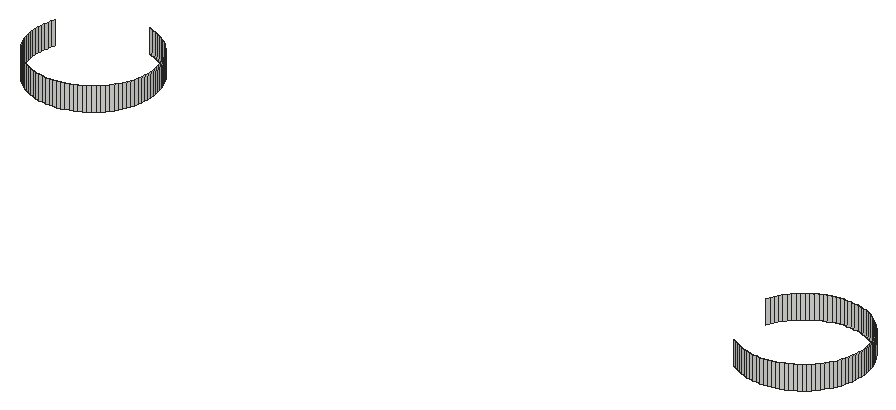
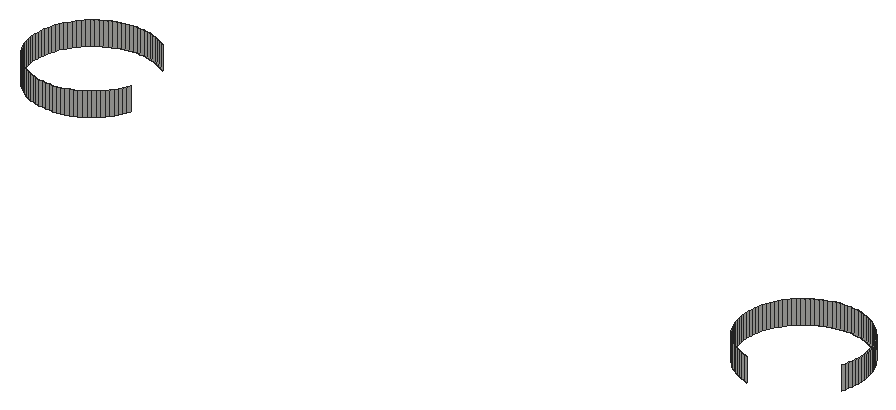
# SketchUp Ruby script. Lengths in inches.
U = 1.inch
M = Sketchup.active_model
def pt(a) = Geom::Point3d.new(a.map { |v| v * U })
def face(e, loops, mat)
  f = e.add_face(loops[0].map { |a| pt(a) })
  loops[1..].each { |l| e.add_face(l.map { |a| pt(a) }).erase! }
  f.material = f.back_material = mat if mat
  f
end
# faces: each face lists its corners as indices into pts; further lists are holes
def faces(e, pts, list, mat = nil) = list.each { |f| face(e, (f[0].is_a?(Array) ? f : [f]).map { |l| l.map { |i| pts[i] } }, mat) }
# xy, xz, yz: faces in a plane at the given z, y or x. An outline is a flat list of corners, or four numbers for a rectangle; further outlines are holes
def ring(l) = l.size == 4 ? [[l[0], l[1]], [l[2], l[1]], [l[2], l[3]], [l[0], l[3]]] : l.each_slice(2).to_a
def flat(e, list, mat, &to3) = list.each { |f| face(e, (f[0].is_a?(Array) ? f : [f]).map { |l| ring(l).map { |u, v| to3.(u, v) } }, mat) }
def xy(e, z, list, mat = nil) = flat(e, list, mat) { |x, y| [x, y, z] }
def xz(e, y, list, mat = nil) = flat(e, list, mat) { |x, z| [x, y, z] }
def yz(e, x, list, mat = nil) = flat(e, list, mat) { |y, z| [x, y, z] }
def lines(e, pts, list) = list.each { |a, b| e.add_line(pt(pts[a]), pt(pts[b])) }
# prism: a flat outline (further loops are holes) pulled along v
def prism(e, loops, v, mat = nil)
  f = face(e, loops, mat); d = Geom::Vector3d.new(v.map { |x| x * U })
  f.pushpull(f.normal.samedirection?(d) ? d.length : -d.length)
end
def box(e, o, s, mat = nil) = prism(e, [[o, [o[0] + s[0], o[1], o[2]], [o[0] + s[0], o[1] + s[1], o[2]], [o[0], o[1] + s[1], o[2]]]], [0, 0, s[2]], mat)
def at(x, y, z, deg = 0) = Geom::Transformation.translation(pt([x, y, z])) * Geom::Transformation.rotation(ORIGIN, Z_AXIS, deg.degrees)
def axes(o, x, y, z) = Geom::Transformation.new([*x, 0, *y, 0, *z, 0, *pt(o).to_a, 1])
def part(name) = M.definitions.add(name)
# library, detail: a bought-in or finely detailed component or shape, given as its bounding box
def library(name, o, s) = part(name).tap { |d| box(d.entities, o, s) }
def detail(e, o, s) = box(e.add_group.entities, o, s)
def put(e, d, t, mat = nil) = e.add_instance(d, t).tap { |i| i.material = mat if mat }
def group(e, t, mat = nil) = e.add_group.tap { |g| g.transformation = t; g.material = mat if mat }.entities
root = M.entities
xz(root,34,[[220.18,231.53,220.56,234],[295.37,231.53,295.75,234]])
xz(root,46,[[295.37,231.53,295.75,234]])
yz(root,214.375,[[39.8125,231.53,40.1875,234]])
yz(root,226.37,[[39.8125,231.53,40.1875,234]])
yz(root,301.56,[[39.8125,231.53,40.1875,234]])
p = [[219.81,34.03,231.53],[219.43,34.07,231.53],[219.43,34.07,234],[219.81,34.03,234],[220.18,34,231.53],[220.18,34,234],
  [220.94,34.03,231.53],[220.56,34,231.53],[220.56,34,234],[220.94,34.03,234],[221.31,34.07,231.53],[221.31,34.07,234],
  [295,34.03,231.53],[294.62,34.07,231.53],[294.62,34.07,234],[295,34.03,234],[295.37,34,231.53],[295.37,34,234],
  [296.125,34.03,231.53],[295.75,34,231.53],[295.75,34,234],[296.125,34.03,234],[296.5,34.07,231.53],[296.5,34.07,234],
  [219.0625,34.14,231.53],[218.7,34.24,231.53],[218.7,34.24,234],[219.0625,34.14,234],[221.68,34.14,231.53],[221.68,34.14,234],
  [222.04,34.24,231.53],[222.04,34.24,234],[294.25,34.14,231.53],[293.89,34.24,231.53],[293.89,34.24,234],[294.25,34.14,234],
  [296.87,34.14,231.53],[296.87,34.14,234],[297.23,34.24,231.53],[297.23,34.24,234],[218.34,34.35,231.53],[218.34,34.35,234],
  [222.4,34.35,231.53],[222.4,34.35,234],[293.53,34.35,231.53],[293.53,34.35,234],[297.59,34.35,231.53],[297.59,34.35,234],
  [217.99,34.49,231.53],[217.99,34.49,234],[222.75,34.49,231.53],[222.75,34.49,234],[293.18,34.49,231.53],[293.18,34.49,234],
  [297.94,34.49,231.53],[297.94,34.49,234],[217.65,34.65,231.53],[217.65,34.65,234],[223.09,34.65,231.53],[223.09,34.65,234],
  [292.84,34.65,231.53],[292.84,34.65,234],[298.28,34.65,231.53],[298.28,34.65,234],[217.32,34.84,231.53],[217.32,34.84,234],
  [223.43,34.84,231.53],[223.43,34.84,234],[292.51,34.84,231.53],[292.51,34.84,234],[298.61,34.84,231.53],[298.61,34.84,234],
  [217,35.04,231.53],[217,35.04,234],[223.74,35.04,231.53],[223.74,35.04,234],[292.1875,35.04,231.53],[292.1875,35.04,234],
  [298.93,35.04,231.53],[298.93,35.04,234],[216.69,35.26,231.53],[216.69,35.26,234],[224.05,35.26,231.53],[224.05,35.26,234],
  [299.24,35.26,231.53],[299.24,35.26,234],[216.4,35.5,231.53],[216.4,35.5,234],[224.34,35.5,231.53],[224.34,35.5,234],
  [299.53,35.5,231.53],[299.53,35.5,234],[216.13,35.76,231.53],[216.13,35.76,234],[224.61,35.76,231.53],[224.61,35.76,234],
  [299.8,35.76,231.53],[299.8,35.76,234],[215.87,36.03,231.53],[215.87,36.03,234],[224.87,36.03,231.53],[224.87,36.03,234],
  [300.0625,36.03,231.53],[300.0625,36.03,234],[215.63,36.32,231.53],[215.63,36.32,234],[225.11,36.32,231.53],[225.11,36.32,234],
  [300.3,36.32,231.53],[300.3,36.32,234],[215.41,36.63,231.53],[215.41,36.63,234],[225.33,36.63,231.53],[225.33,36.63,234],
  [300.52,36.63,231.53],[300.52,36.63,234],[215.21,36.95,231.53],[215.21,36.95,234],[225.54,36.95,231.53],[225.54,36.95,234],
  [300.72,36.95,231.53],[300.72,36.95,234],[215.02,37.28,231.53],[215.02,37.28,234],[225.72,37.28,231.53],[225.72,37.28,234],
  [300.91,37.28,231.53],[300.91,37.28,234],[214.86,37.62,231.53],[214.86,37.62,234],[225.88,37.62,231.53],[225.88,37.62,234],
  [301.07,37.62,231.53],[301.07,37.62,234],[214.73,37.97,231.53],[214.73,37.97,234],[226.02,37.97,231.53],[226.02,37.97,234],
  [301.21,37.97,231.53],[301.21,37.97,234],[214.61,38.33,231.53],[214.61,38.33,234],[226.13,38.33,231.53],[226.13,38.33,234],
  [301.32,38.33,231.53],[301.32,38.33,234],[214.52,38.69,231.53],[214.52,38.69,234],[226.23,38.69,231.53],[226.23,38.69,234],
  [301.42,38.69,231.53],[301.42,38.69,234],[214.44,39.0625,231.53],[214.44,39.0625,234],[226.3,39.0625,231.53],[226.3,39.0625,234],
  [301.49,39.0625,231.53],[301.49,39.0625,234],[214.4,39.44,231.53],[214.4,39.44,234],[226.34,39.44,231.53],[226.34,39.44,234],
  [301.53,39.44,231.53],[301.53,39.44,234],[214.375,39.8125,231.53],[214.375,39.8125,234],[226.37,39.8125,231.53],[226.37,39.8125,234],
  [301.56,39.8125,231.53],[301.56,39.8125,234],[214.375,40.1875,231.53],[214.4,40.56,231.53],[214.4,40.56,234],[214.375,40.1875,234],
  [226.34,40.56,231.53],[226.37,40.1875,231.53],[226.37,40.1875,234],[226.34,40.56,234],[301.53,40.56,231.53],[301.56,40.1875,231.53],
  [301.56,40.1875,234],[301.53,40.56,234],[214.44,40.9375,231.53],[214.44,40.9375,234],[226.3,40.9375,231.53],[226.3,40.9375,234],
  [301.49,40.9375,231.53],[301.49,40.9375,234],[214.52,41.31,231.53],[214.52,41.31,234],[226.23,41.31,231.53],[226.23,41.31,234],
  [301.42,41.31,231.53],[301.42,41.31,234],[214.61,41.67,231.53],[214.61,41.67,234],[226.13,41.67,231.53],[226.13,41.67,234],
  [301.32,41.67,231.53],[301.32,41.67,234],[214.73,42.03,231.53],[214.73,42.03,234],[226.02,42.03,231.53],[226.02,42.03,234],
  [301.21,42.03,231.53],[301.21,42.03,234],[225.88,42.38,231.53],[225.88,42.38,234],[289.92,42.03,231.53],[290.05,42.38,231.53],
  [290.05,42.38,234],[289.92,42.03,234],[301.07,42.38,231.53],[301.07,42.38,234],[225.72,42.72,231.53],[225.72,42.72,234],
  [290.21,42.72,231.53],[290.21,42.72,234],[300.91,42.72,231.53],[300.91,42.72,234],[225.54,43.05,231.53],[225.54,43.05,234],
  [290.4,43.05,231.53],[290.4,43.05,234],[300.72,43.05,231.53],[300.72,43.05,234],[225.33,43.37,231.53],[225.33,43.37,234],
  [290.6,43.37,231.53],[290.6,43.37,234],[300.52,43.37,231.53],[300.52,43.37,234],[225.11,43.68,231.53],[225.11,43.68,234],
  [290.82,43.68,231.53],[290.82,43.68,234],[300.3,43.68,231.53],[300.3,43.68,234],[224.87,43.97,231.53],[224.87,43.97,234],
  [291.06,43.97,231.53],[291.06,43.97,234],[300.0625,43.97,231.53],[300.0625,43.97,234],[224.61,44.24,231.53],[224.61,44.24,234],
  [291.32,44.24,231.53],[291.32,44.24,234],[299.8,44.24,231.53],[299.8,44.24,234],[224.34,44.5,231.53],[224.34,44.5,234],
  [291.59,44.5,231.53],[291.59,44.5,234],[299.53,44.5,231.53],[299.53,44.5,234],[224.05,44.74,231.53],[224.05,44.74,234],
  [291.88,44.74,231.53],[291.88,44.74,234],[299.24,44.74,231.53],[299.24,44.74,234],[223.74,44.96,231.53],[223.74,44.96,234],
  [292.1875,44.96,231.53],[292.1875,44.96,234],[298.93,44.96,231.53],[298.93,44.96,234],[223.43,45.16,231.53],[223.43,45.16,234],
  [292.51,45.16,231.53],[292.51,45.16,234],[298.61,45.16,231.53],[298.61,45.16,234],[223.09,45.35,231.53],[223.09,45.35,234],
  [292.84,45.35,231.53],[292.84,45.35,234],[298.28,45.35,231.53],[298.28,45.35,234],[222.75,45.51,231.53],[222.75,45.51,234],
  [293.18,45.51,231.53],[293.18,45.51,234],[297.94,45.51,231.53],[297.94,45.51,234],[222.4,45.65,231.53],[222.4,45.65,234],
  [293.53,45.65,231.53],[293.53,45.65,234],[297.59,45.65,231.53],[297.59,45.65,234],[222.04,45.76,231.53],[222.04,45.76,234],
  [293.89,45.76,231.53],[293.89,45.76,234],[297.23,45.76,231.53],[297.23,45.76,234],[221.68,45.86,231.53],[221.68,45.86,234],
  [294.25,45.86,231.53],[294.25,45.86,234],[296.87,45.86,231.53],[296.87,45.86,234],[294.62,45.93,231.53],[294.62,45.93,234],
  [295,45.97,231.53],[295,45.97,234],[296.125,45.97,231.53],[296.5,45.93,231.53],[296.5,45.93,234],[296.125,45.97,234],
  [295.37,46,231.53],[295.37,46,234],[295.75,46,231.53],[295.75,46,234]]
faces(root,p,[[0,1,2,3],[4,0,3,5],[6,7,8,9],[10,6,9,11],[12,13,14,15],[16,12,15,17],[18,19,20,21],[22,18,21,23],
  [24,25,26,27],[1,24,27,2],[28,10,11,29],[30,28,29,31],[32,33,34,35],[13,32,35,14],[36,22,23,37],[38,36,37,39],
  [25,40,41,26],[42,30,31,43],[33,44,45,34],[46,38,39,47],[40,48,49,41],[50,42,43,51],[44,52,53,45],[54,46,47,55],
  [48,56,57,49],[58,50,51,59],[52,60,61,53],[62,54,55,63],[56,64,65,57],[66,58,59,67],[60,68,69,61],[70,62,63,71],
  [64,72,73,65],[74,66,67,75],[68,76,77,69],[78,70,71,79],[72,80,81,73],[82,74,75,83],[84,78,79,85],[80,86,87,81],
  [88,82,83,89],[90,84,85,91],[86,92,93,87],[94,88,89,95],[96,90,91,97],[92,98,99,93],[100,94,95,101],[102,96,97,103],
  [98,104,105,99],[106,100,101,107],[108,102,103,109],[104,110,111,105],[112,106,107,113],[114,108,109,115],[110,116,117,111],[118,112,113,119],
  [120,114,115,121],[116,122,123,117],[124,118,119,125],[126,120,121,127],[122,128,129,123],[130,124,125,131],[132,126,127,133],[128,134,135,129],
  [136,130,131,137],[138,132,133,139],[134,140,141,135],[142,136,137,143],[144,138,139,145],[140,146,147,141],[148,142,143,149],[150,144,145,151],
  [146,152,153,147],[154,148,149,155],[156,150,151,157],[152,158,159,153],[160,154,155,161],[162,156,157,163],[158,164,165,159],[166,160,161,167],
  [168,162,163,169],[170,171,172,173],[174,175,176,177],[178,179,180,181],[171,182,183,172],[184,174,177,185],[186,178,181,187],[182,188,189,183],
  [190,184,185,191],[192,186,187,193],[188,194,195,189],[196,190,191,197],[198,192,193,199],[194,200,201,195],[202,196,197,203],[204,198,199,205],
  [206,202,203,207],[208,209,210,211],[212,204,205,213],[214,206,207,215],[209,216,217,210],[218,212,213,219],[220,214,215,221],[216,222,223,217],
  [224,218,219,225],[226,220,221,227],[222,228,229,223],[230,224,225,231],[232,226,227,233],[228,234,235,229],[236,230,231,237],[238,232,233,239],
  [234,240,241,235],[242,236,237,243],[244,238,239,245],[240,246,247,241],[248,242,243,249],[250,244,245,251],[246,252,253,247],[254,248,249,255],
  [256,250,251,257],[252,258,259,253],[260,254,255,261],[262,256,257,263],[258,264,265,259],[266,260,261,267],[268,262,263,269],[264,270,271,265],
  [272,266,267,273],[274,268,269,275],[270,276,277,271],[278,272,273,279],[280,274,275,281],[276,282,283,277],[284,278,279,285],[286,280,281,287],
  [282,288,289,283],[290,284,285,291],[292,286,287,293],[288,294,295,289],[296,290,291,297],[298,292,293,299],[294,300,301,295],[302,296,297,303],
  [300,304,305,301],[304,306,307,305],[308,309,310,311],[309,302,303,310],[306,312,313,307],[314,308,311,315]])
